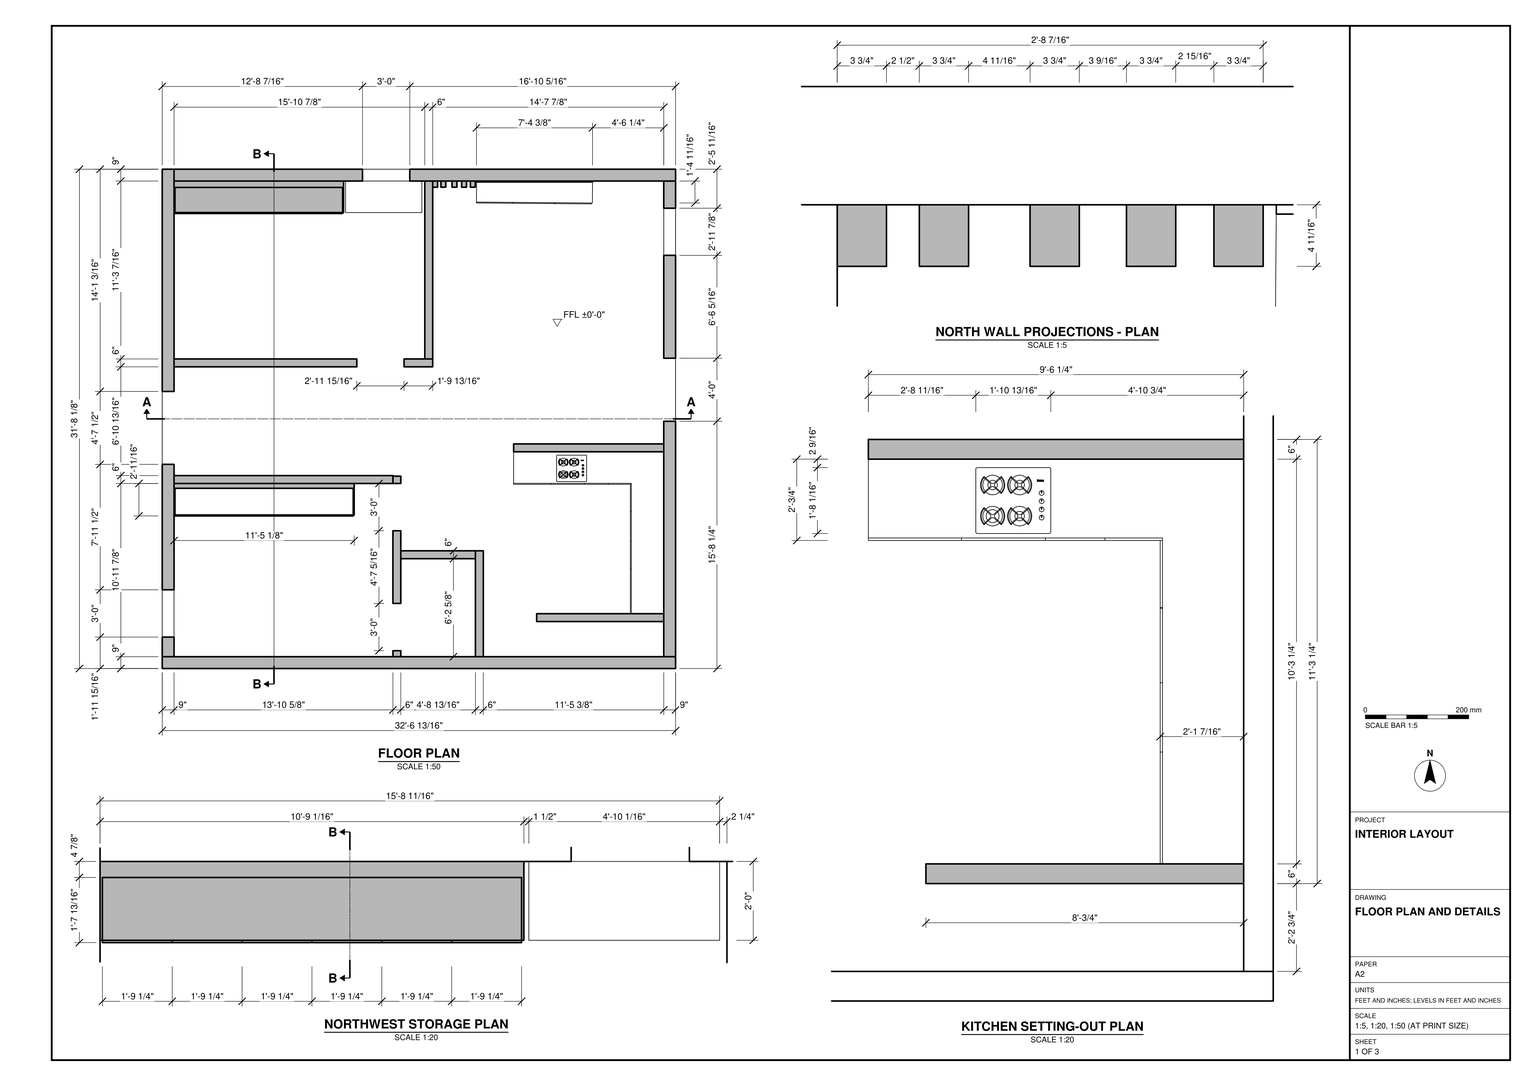
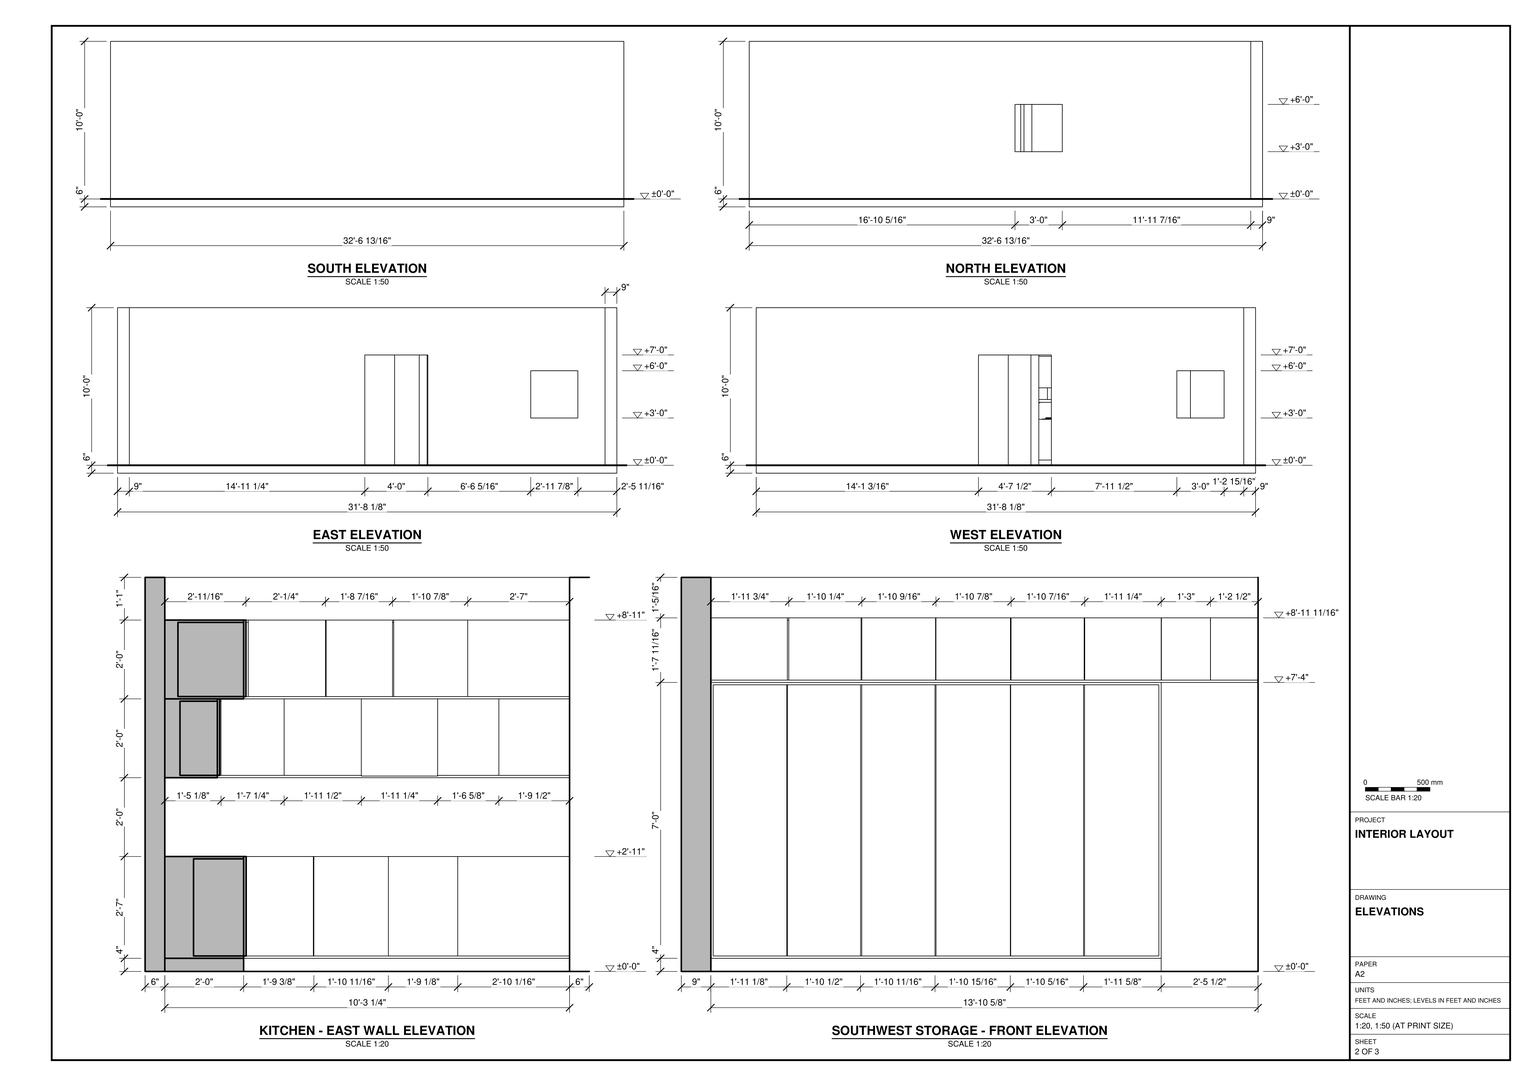
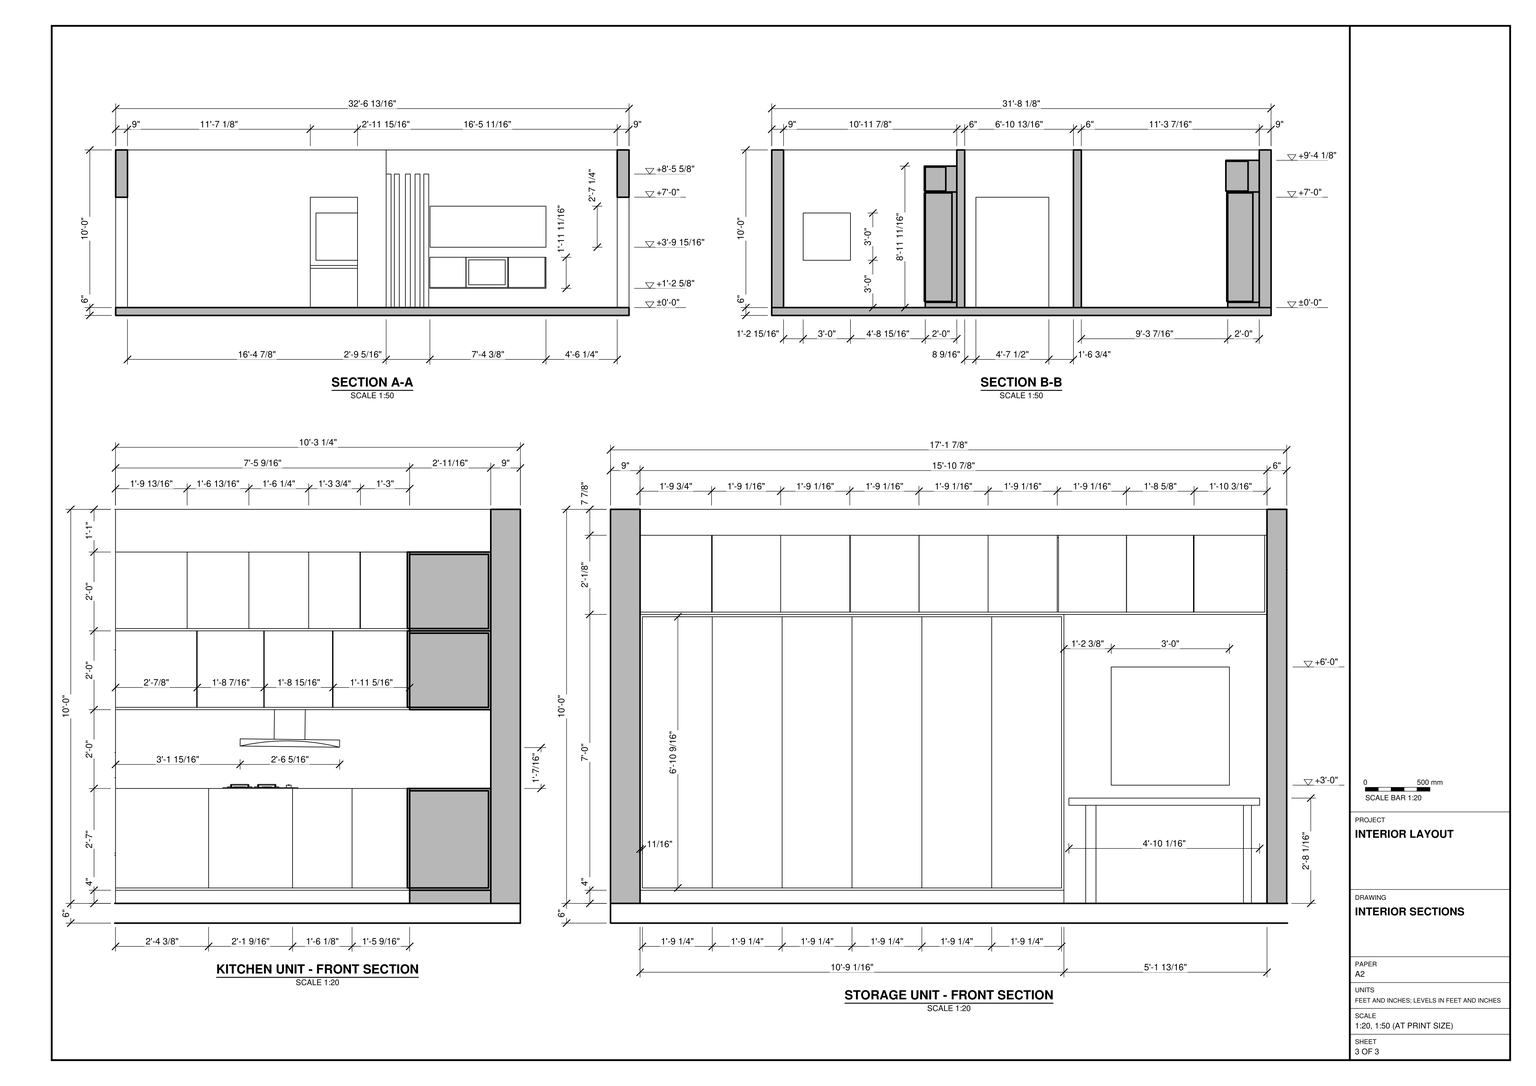
Build the interior in SketchUp from task_files/diagram_01.pdf. Work in feet and inches. Set the finished floor at ±0'-0". The overall dimensions are 32'-6 13/16" east to west, 31'-8 1/8" north to south and 10'-6" high, including the 6" floor slab below the finished floor.

Lay out the 9" perimeter walls and 6" interior partitions from the floor plan. Preserve the passage between the east and west doorway openings and the gaps that connect it to the rooms. Use the exterior elevations to set the window sills and heads; the south wall is uninterrupted.

Fit the northwest room with tall divided storage and a table beneath the window, with overhead cupboards extending across both. Build the southwest storage with its shorter bank of tall cupboards and longer overhead row. In the southeast kitchen, turn the worktop and cabinetry along the east wall. Follow the kitchen elevations for the plinths, cabinet divisions and two rows of upper cupboards. Place the cooktop on the transverse run with the extractor above it. On the north wall, use the projection detail and section A-A to position the vertical projections beside the raised cabinet and panel.

Keep shell elements and each furniture or joinery piece in separate groups or components, and use components for repeated parts. Decor, loose items and appliances may be any suitable library components. Save one SketchUp model as output_files/interior_with_fitted_storage_and_an_l_shaped_kitchen.skp.

# SketchUp Ruby script. Lengths in inches.
U = 1.inch
M = Sketchup.active_model
def pt(a) = Geom::Point3d.new(a.map { |v| v * U })
def face(e, loops, mat)
  f = e.add_face(loops[0].map { |a| pt(a) })
  loops[1..].each { |l| e.add_face(l.map { |a| pt(a) }).erase! }
  f.material = f.back_material = mat if mat
  f
end
# faces: each face lists its corners as indices into pts; further lists are holes
def faces(e, pts, list, mat = nil) = list.each { |f| face(e, (f[0].is_a?(Array) ? f : [f]).map { |l| l.map { |i| pts[i] } }, mat) }
# xy, xz, yz: faces in a plane at the given z, y or x. An outline is a flat list of corners, or four numbers for a rectangle; further outlines are holes
def ring(l) = l.size == 4 ? [[l[0], l[1]], [l[2], l[1]], [l[2], l[3]], [l[0], l[3]]] : l.each_slice(2).to_a
def flat(e, list, mat, &to3) = list.each { |f| face(e, (f[0].is_a?(Array) ? f : [f]).map { |l| ring(l).map { |u, v| to3.(u, v) } }, mat) }
def xy(e, z, list, mat = nil) = flat(e, list, mat) { |x, y| [x, y, z] }
def xz(e, y, list, mat = nil) = flat(e, list, mat) { |x, z| [x, y, z] }
def yz(e, x, list, mat = nil) = flat(e, list, mat) { |y, z| [x, y, z] }
def lines(e, pts, list) = list.each { |a, b| e.add_line(pt(pts[a]), pt(pts[b])) }
# prism: a flat outline (further loops are holes) pulled along v
def prism(e, loops, v, mat = nil)
  f = face(e, loops, mat); d = Geom::Vector3d.new(v.map { |x| x * U })
  f.pushpull(f.normal.samedirection?(d) ? d.length : -d.length)
end
def box(e, o, s, mat = nil) = prism(e, [[o, [o[0] + s[0], o[1], o[2]], [o[0] + s[0], o[1] + s[1], o[2]], [o[0], o[1] + s[1], o[2]]]], [0, 0, s[2]], mat)
def at(x, y, z, deg = 0) = Geom::Transformation.translation(pt([x, y, z])) * Geom::Transformation.rotation(ORIGIN, Z_AXIS, deg.degrees)
def axes(o, x, y, z) = Geom::Transformation.new([*x, 0, *y, 0, *z, 0, *pt(o).to_a, 1])
def part(name) = M.definitions.add(name)
# library, detail: a bought-in or finely detailed component or shape, given as its bounding box
def library(name, o, s) = part(name).tap { |d| box(d.entities, o, s) }
def detail(e, o, s) = box(e.add_group.entities, o, s)
def put(e, d, t, mat = nil) = e.add_instance(d, t).tap { |i| i.material = mat if mat }
def group(e, t, mat = nil) = e.add_group.tap { |g| g.transformation = t; g.material = mat if mat }.entities
root = M.entities
M.materials.add("[0011_Seashell]").color = [255, 245, 238]
M.materials.add("[0014_DarkSalmon]").color = [233, 150, 122]
M.materials.add("[Wood Floor]").color = [155, 105, 61]
M.materials.add("[Wood Veneer 01]").color = [120, 70, 37]
c1 = library("1-TABLE DE CUISSON CLC2",[-11.42,-10.04,0],[22.84,20.08,1.26])
c2 = library("5-HOTTE ASPIRANTE CLC2",[-15.16,-17.72,-0.29],[30.34,17.72,30.09])
c3 = part("Group\#44")
box(c3.entities,[0,0,0],[21.27,0.71,82.58])
c4 = part("Group\#45")
box(c4.entities,[0,0,0],[21.27,0.71,82.58])
c5 = part("Group\#62")
box(c5.entities,[0,-4.6875,0],[3.75,4.6875,101.64])
box(root,[356.38,119.78,4.71],[0.71,20.45,30.29])
box(root,[267.52,148.29,59.71],[24.71,0.71,23.29])
box(root,[326.36,140.29,83.71],[15.59,0.71,23.29])
box(root,[9,116.17,88.71],[23.29,0.71,18.97])
xy(root,4.71,[[9.71,116.17,32.11,116.88],[32.33,116.17,54.58,116.88],[54.94,116.17,77.25,116.88],[77.5625,116.17,100.18,116.88],[100.31,116.17,122.48,116.88],
  [122.8,116.17,145.42,116.88]])
xy(root,87.29,[[9.71,116.17,32.11,116.88],[32.33,116.17,54.58,116.88],[54.94,116.17,77.25,116.88],[77.5625,116.17,100.18,116.88],[100.31,116.17,122.48,116.88],
  [122.8,116.17,145.42,116.88]])
xy(root,88.71,[[9,345.71,30.76,346.42],[30.98,345.71,51.82,346.42],[51.82,345.71,72.87,346.42],[73.01,345.71,93.92,346.42],[93.97,345.71,114.98,346.42],
  [114.98,345.71,136.03,346.42],[136.41,345.71,157.08,346.42],[157.15,345.71,177.5,346.42],[177.7,345.71,199.19,346.42]])
xy(root,112.1,[[9,345.71,30.76,346.42],[30.98,345.71,51.82,346.42],[51.82,345.71,72.87,346.42],[73.01,345.71,93.92,346.42],[93.97,345.71,114.98,346.42],
  [114.98,345.71,136.03,346.42],[136.41,345.71,157.08,346.42],[157.15,345.71,177.5,346.42],[177.7,345.71,199.19,346.42]])
xz(root,116.17,[[9.71,4.71,32.11,87.29],[32.33,4.71,54.58,87.29],[54.94,4.71,77.25,87.29],[77.5625,4.71,100.18,87.29],[100.31,4.71,122.48,87.29],
  [122.8,4.71,145.42,87.29]],"[Wood Veneer 01]")
xz(root,116.88,[[9.71,4.71,32.11,87.29],[32.33,4.71,54.58,87.29],[54.94,4.71,77.25,87.29],[77.5625,4.71,100.18,87.29],[100.31,4.71,122.48,87.29],
  [122.8,4.71,145.42,87.29]])
xz(root,345.71,[[9,88.71,30.76,112.1],[30.98,88.71,51.82,112.1],[51.82,88.71,72.87,112.1],[73.01,88.71,93.92,112.1],[93.97,88.71,114.98,112.1],
  [114.98,88.71,136.03,112.1],[136.41,88.71,157.08,112.1],[157.15,88.71,177.5,112.1],[177.7,88.71,199.19,112.1]],"[0011_Seashell]")
xz(root,346.42,[[9,88.71,30.76,112.1],[30.98,88.71,51.82,112.1],[51.82,88.71,72.87,112.1],[93.97,88.71,114.98,112.1],[114.98,88.71,136.03,112.1],
  [177.7,88.71,199.19,112.1]])
yz(root,9,[[345.71,88.71,346.42,112.1]])
yz(root,9.71,[[116.17,4.71,116.88,87.29]])
yz(root,30.76,[[345.71,88.71,346.42,111.39],[345.71,111.39,346.42,112.1]])
yz(root,30.98,[[345.71,88.71,346.42,112.1]])
yz(root,32.11,[[116.17,4.71,116.88,87.29]])
yz(root,32.33,[[116.17,4.71,116.88,87.29]])
yz(root,51.82,[[345.71,88.71,346.42,112.1]])
yz(root,54.58,[[116.17,4.71,116.88,87.29]])
yz(root,54.94,[[116.17,4.71,116.88,87.29]])
yz(root,72.87,[[345.71,88.71,346.42,112.1]])
yz(root,73.01,[[345.71,88.71,346.42,112.1]])
yz(root,77.25,[[116.17,4.71,116.88,87.29]])
yz(root,77.5625,[[116.17,4.71,116.88,87.29]])
yz(root,93.92,[[345.71,88.71,346.42,112.1]])
yz(root,93.97,[[345.71,88.71,346.42,112.1]])
yz(root,100.18,[[116.17,4.71,116.88,87.29]])
yz(root,100.31,[[116.17,4.71,116.88,87.29]])
yz(root,114.98,[[345.71,88.71,346.42,112.1]])
yz(root,122.48,[[116.17,4.71,116.88,87.29]])
yz(root,122.8,[[116.17,4.71,116.88,87.29]])
yz(root,136.03,[[345.71,88.71,346.42,112.1]])
yz(root,136.41,[[345.71,88.71,346.42,112.1]])
yz(root,145.42,[[116.17,4.71,116.88,87.29]])
yz(root,157.08,[[345.71,88.71,346.42,112.1]])
yz(root,157.15,[[345.71,88.71,346.42,112.1]])
yz(root,177.5,[[345.71,88.71,346.42,112.1]])
yz(root,177.7,[[345.71,88.71,346.42,112.1]])
yz(root,199.19,[[345.71,88.71,346.42,112.1]])
p = [[9.71,346.42,111.39],[30.76,346.42,111.39],[30.98,346.42,111.39],[72.87,346.42,111.39],[73.01,346.42,111.39],[93.92,346.42,111.39],
  [93.97,346.42,111.39],[136.03,346.42,111.39],[136.41,346.42,111.39],[157.08,346.42,111.39],[157.15,346.42,111.39],[177.5,346.42,111.39],
  [177.7,346.42,111.39],[100.18,116.88,87.29],[100.31,116.88,87.29],[122.48,116.88,87.29],[122.8,116.88,87.29],[77.25,116.88,87.29],
  [77.5625,116.88,87.29],[54.58,116.88,87.29],[54.94,116.88,87.29],[32.11,116.88,87.29],[32.33,116.88,87.29]]
lines(root,p,[[0,1],[1,2],[3,4],[5,6],[7,8],[9,10],[11,12],[13,14],[15,16],[17,18],[19,20],[21,22]])
put(root,c1,at(311.65,152.39,35))
put(root,c2,axes([320.6,166.01,47.75],[0.99919,0,0],[0,1,0],[0,0,1]))
g1 = group(root,at(0,0,0))
box(g1,[0,0,0],[390.8,9,120])
g2 = group(root,at(0,9,0))
prism(g2,[[[0,371.125,0],[0,201.9375,0],[0,201.9375,84],[0,146.4375,84],[0,146.4375,0],[0,0,0],[0,0,120],[0,371.125,120]],[[0,50.9375,72],[0,14.9375,72],[0,14.9375,36],[0,50.9375,36]]],[9,0,0])
g3 = group(root,at(175.625,9,0))
prism(g3,[[[6,0,0],[6,4.57,0],[6,4.57,84],[6,40.57,84],[6,40.57,0],[6,95.88,0],[6,95.88,84],[6,131.88,84],[6,131.88,0],[6,137.45,0],[6,137.45,120],[6,0,120]]],[-6,0,0])
g4 = group(root,at(9,140.88,0))
box(g4,[0,0,0],[166.625,6,120])
g5 = group(root,at(238.43,9,0))
box(g5,[0,0,0],[6,80.625,120])
g6 = group(root,at(181.625,83.625,0))
box(g6,[0,0,0],[56.8,6,120])
g7 = group(root,at(381.8,9,0))
prism(g7,[[[9,0,0],[9,179.25,0],[9,179.25,84],[9,227.25,84],[9,227.25,0],[9,362.125,0],[9,362.125,120],[9,0,120]],[[9,305.5625,36],[9,305.5625,72],[9,341.4375,72],[9,341.4375,36]]],[-9,0,0])
g8 = group(root,at(9,371.125,0))
prism(g8,[[[0,0,0],[381.8,0,0],[381.8,0,120],[0,0,120]],[[179.46,0,72],[179.46,0,36],[143.46,0,36],[143.46,0,72]]],[0,9,0])
g9 = group(root,at(267.52,165,0))
box(g9,[0,0,0],[114.28,6,120])
g10 = group(root,at(199.9,235.68,0))
box(g10,[0,0,0],[6,135.45,120])
g11 = group(root,at(9,229.68,0))
prism(g11,[[[0,0,0],[139.15,0,0],[139.15,0,84],[175.1,0,84],[175.1,0,0],[196.9,0,0],[196.9,0,120],[0,0,120]]],[0,6,0])
g12 = group(root,at(0,0,-6))
box(g12,[0,0,0],[390.8,380.125,6])
g13 = group(root,at(285.05,35.75,0))
box(g13,[0,0,0],[96.75,6,120])
g14 = group(root,at(267.52,141,0))
prism(g14,[[[114.28,24,0],[114.28,-99.25,0],[89.57,-99.25,0],[89.57,0,0],[0,0,0],[0,24,0]]],[0,0,4])
g15 = group(root,at(267.52,141,4))
xy(g15,0,[[89.57,-99.25,89.57,0,0,0,0,24,114.28,24,114.28,-99.25]])
xy(g15,0.71,[[89.57,-99.25,113.57,-99.25,113.57,15.25,0.71,15.25,0.71,0,89.57,0]])
xy(g15,30.29,[[89.57,-99.25,89.57,0,0.71,0,0.71,15.25,113.57,15.25,113.57,-99.25]])
xy(g15,31,[[89.57,-99.25,114.28,-99.25,114.28,24,0,24,0,0,89.57,0]])
xz(g15,-99.25,[[89.57,0,114.28,0,114.28,31,89.57,31,89.57,30.29,113.57,30.29,113.57,0.71,89.57,0.71]])
xz(g15,0,[[0,0,89.57,0,89.57,0.71,0.71,0.71,0.71,30.29,89.57,30.29,89.57,31,0,31]])
xz(g15,15.25,[[0.71,0.71,113.57,30.29]])
xz(g15,24,[[0,0,114.28,31]])
yz(g15,0,[[0,0,24,31]])
yz(g15,0.71,[[0,0.71,15.25,30.29]])
yz(g15,89.57,[[-99.25,0,0,0.71],[-99.25,30.29,0,31]])
yz(g15,113.57,[[-99.25,0.71,15.25,30.29]])
yz(g15,114.28,[[-99.25,0,24,31]])
g16 = group(root,at(267.52,140.23,4.71))
box(g16,[0,0,0],[28.35,0.77,30.29])
g17 = group(root,at(295.87,140.23,4.71))
box(g17,[0,0,0],[25.5625,0.77,30.29])
g18 = group(root,at(321.43,140.23,4.71))
box(g18,[0,0,0],[18.125,0.77,30.29])
g19 = group(root,at(339.56,140.23,4.71))
box(g19,[0,0,0],[17.53,0.77,30.29])
g20 = group(root,at(356.38,96.92,4.71))
box(g20,[0,0,0],[0.71,22.69,30.29])
g21 = group(root,at(356.38,75.8,4.71))
box(g21,[0,0,0],[0.71,21.11,30.29])
g22 = group(root,at(356.38,41.75,4.71))
box(g22,[0,0,0],[0.71,34.05,30.29])
g23 = group(root,at(267.52,165,59))
xy(g23,0,[[89.57,-123.25,89.57,-16,0,-16,0,0,114.28,0,114.28,-123.25]])
xy(g23,0.71,[[89.57,-123.25,113.57,-123.25,113.57,-4.625,0.71,-4.625,0.71,-16,89.57,-16]])
xy(g23,23.29,[[89.57,-123.25,89.57,-16,0.71,-16,0.71,-4.625,113.57,-4.625,113.57,-123.25]])
xy(g23,24,[[89.57,-123.25,114.28,-123.25,114.28,0,0,0,0,-16,89.57,-16]])
xz(g23,-123.25,[[89.57,0,114.28,0,114.28,24,89.57,24,89.57,23.29,113.57,23.29,113.57,0.71,89.57,0.71]])
xz(g23,-16,[[0,0,89.57,0,89.57,0.71,0.71,0.71,0.71,23.29,89.57,23.29,89.57,24,0,24]])
xz(g23,-4.625,[[0.71,0.71,113.57,23.29]])
xz(g23,0,[[0,0,114.28,24]])
yz(g23,0,[[-16,0,0,24]])
yz(g23,0.71,[[-16,0.71,-4.625,23.29]])
yz(g23,89.57,[[-123.25,0,-16,0.71],[-123.25,23.29,-16,24]])
yz(g23,113.57,[[-123.25,0.71,-4.625,23.29]])
yz(g23,114.28,[[-123.25,0,0,24]])
g24 = group(root,at(292.41,148.29,59.71))
box(g24,[0,0,0],[20.25,0.71,23.29])
g25 = group(root,at(312.82,148.29,59.71))
box(g25,[0,0,0],[20.76,0.71,23.29])
g26 = group(root,at(333.77,148.29,59.71))
box(g26,[0,0,0],[23.32,0.71,23.29])
g27 = group(root,at(356.38,128.66,59.71))
box(g27,[0,0,0],[0.71,19.22,23.29])
g28 = group(root,at(356.38,105.17,59.71))
box(g28,[0,0,0],[0.71,23.5,23.29])
g29 = group(root,at(356.38,81.92,59))
box(g29,[0,0,0.5],[0.71,23.25,23.5])
g30 = group(root,at(356.38,63.28,59.71))
box(g30,[0,0,0],[0.71,18.64,23.29])
g31 = group(root,at(356.38,41.75,59.71))
box(g31,[0,0,0],[0.71,21.53,23.29])
g32 = group(root,at(267.52,165,83))
xy(g32,0,[[89.57,-123.25,89.57,-24,0,-24,0,0,114.28,0,114.28,-123.25]])
xy(g32,0.71,[[89.57,-123.25,113.57,-123.25,113.57,-4,0.71,-4,0.71,-24,89.57,-24]])
xy(g32,23.29,[[89.57,-123.25,89.57,-24,0.71,-24,0.71,-4,113.57,-4,113.57,-123.25]])
xy(g32,24,[[89.57,-123.25,114.28,-123.25,114.28,0,0,0,0,-24,89.57,-24]])
xz(g32,-123.25,[[89.57,0,114.28,0,114.28,24,89.57,24,89.57,23.29,113.57,23.29,113.57,0.71,89.57,0.71]])
xz(g32,-24,[[0,0,89.57,0,89.57,0.71,0.71,0.71,0.71,23.29,89.57,23.29,89.57,24,0,24]])
xz(g32,-4,[[0.71,0.71,113.57,23.29]])
xz(g32,0,[[0,0,114.28,24]])
yz(g32,0,[[-24,0,0,24]])
yz(g32,0.71,[[-24,0.71,-4,23.29]])
yz(g32,89.57,[[-123.25,0,-24,0.71],[-123.25,23.29,-24,24]])
yz(g32,113.57,[[-123.25,0.71,-4,23.29]])
yz(g32,114.28,[[-123.25,0,0,24]])
g33 = group(root,at(267.52,140.29,83.71))
box(g33,[0,0,0],[21.81,0.71,23.29])
g34 = group(root,at(289.34,140.29,83.71))
box(g34,[0,0,0],[18.8,0.71,23.29])
g35 = group(root,at(308.13,140.29,83.71))
box(g35,[0,0,0],[18.22,0.71,23.29])
g36 = group(root,at(342.49,140.29,83.71))
box(g36,[-0.375,0,0],[14.98,0.71,23.29])
g37 = group(root,at(356.38,116.07,83.71))
box(g37,[0,0,0],[0.71,23.53,23.29])
g38 = group(root,at(356.38,95.65,83.71))
box(g38,[0,0,0],[0.71,20.21,23.29])
g39 = group(root,at(356.38,76.76,83.71))
box(g39,[0,-4,0],[0.71,22.53,23.29])
g40 = group(root,at(356.38,41.75,83.71))
box(g40,[0,0,0],[0.71,31.01,23.29])
g41 = group(root,at(9,347.125,0))
box(g41,[0,0,0],[129.0625,24,4])
g42 = group(root,at(9,347.125,4))
xy(g42,0,[[0,0,129.0625,24]])
xy(g42,0.71,[[0.71,0,128.35,19.125]])
xy(g42,83.29,[[0.71,0,128.35,19.125]])
xy(g42,84,[[0,0,129.0625,24]])
xz(g42,0,[[[0,0,129.0625,84],[0.71,0.71,128.35,83.29]]])
xz(g42,19.125,[[0.71,0.71,128.35,83.29]])
xz(g42,24,[[0,0,129.0625,84]])
yz(g42,0,[[0,0,24,84]])
yz(g42,0.71,[[0,0.71,19.125,83.29]])
yz(g42,128.35,[[0,0.71,19.125,83.29]])
yz(g42,129.0625,[[0,0,24,84]])
put(root,c3,at(116.08,346.42,4.71),"[0014_DarkSalmon]")
put(root,c3,at(94.81,346.42,4.71),"[0014_DarkSalmon]")
put(root,c3,at(73.53,346.42,4.71),"[0014_DarkSalmon]")
put(root,c4,at(52.26,346.42,4.71),"[0014_DarkSalmon]")
put(root,c4,at(30.98,346.42,4.71),"[0014_DarkSalmon]")
put(root,c4,at(9.71,346.42,4.71),"[0014_DarkSalmon]")
g43 = group(root,at(9,371.125,88))
xy(g43,0,[[0,-24.71,190.9,0]])
xy(g43,0.71,[[0.71,-24.71,190.19,-8.52]])
xy(g43,23.39,[[0.71,-24.71,190.19,-8.52]])
xy(g43,24.1,[[0,-24.71,190.9,0]])
xz(g43,-24.71,[[[0,0,190.9,24.1],[0.71,0.71,190.19,23.39]]])
xz(g43,-8.52,[[0.71,0.71,190.19,23.39]])
xz(g43,0,[[0,0,190.9,24.1]])
yz(g43,0,[[-24.71,0,0,24.1]])
yz(g43,0.71,[[-24.71,0.71,-8.52,23.39]])
yz(g43,190.19,[[-24.71,0.71,-8.52,23.39]])
yz(g43,190.9,[[-24.71,0,0,24.1]])
g44 = group(root,at(139.58,371.125,29.875),"[Wood Veneer 01]")
xy(g44,0,[[0,-24,58.09,0]],"[Wood Floor]")
xy(g44,2.1875,[[0,-24,58.09,0]],"[Wood Veneer 01]")
xz(g44,-24,[[0,0,58.09,2.1875]],"[Wood Veneer 01]")
xz(g44,0,[[0,0,58.09,2.1875]],"[Wood Floor]")
yz(g44,0,[[-24,0,0,2.1875]],"[Wood Floor]")
yz(g44,58.09,[[-24,0,0,2.1875]],"[Wood Floor]")
g45 = group(root,at(9,116.88,0))
box(g45,[0,0,0],[137.125,24,4])
g46 = group(root,at(9,116.88,4))
xy(g46,0,[[0,0,137.125,24]])
xy(g46,0.71,[[0.71,0,136.42,20.3125]])
xy(g46,83.29,[[0.71,0,136.42,20.3125]])
xy(g46,84,[[0,0,137.125,24]])
xz(g46,0,[[[0,0,137.125,84],[0.71,0.71,136.42,83.29]]])
xz(g46,20.3125,[[0.71,0.71,136.42,83.29]])
xz(g46,24,[[0,0,137.125,84]])
yz(g46,0,[[0,0,24,84]])
yz(g46,0.71,[[0,0.71,20.3125,83.29]])
yz(g46,136.42,[[0,0.71,20.3125,83.29]])
yz(g46,137.125,[[0,0,24,84]])
g47 = group(root,at(9,140.88,88))
xy(g47,0,[[0,-24,166.625,0]])
xy(g47,0.71,[[0.71,-24,165.92,-8.375]])
xy(g47,18.97,[[0.71,-24,165.92,-8.375]])
xy(g47,19.68,[[0,-24,166.625,0]])
xz(g47,-24,[[[0,0,166.625,19.68],[0.71,0.71,165.92,18.97]]])
xz(g47,-8.375,[[0.71,0.71,165.92,18.97]])
xz(g47,0,[[0,0,166.625,19.68]])
yz(g47,0,[[-24,0,0,19.68]])
yz(g47,0.71,[[-24,0.71,-8.375,18.97]])
yz(g47,165.92,[[-24,0.71,-8.375,18.97]])
yz(g47,166.625,[[-24,0,0,19.68]])
g48 = group(root,at(32.73,116.17,88.71))
box(g48,[0,0,0],[22,0.71,18.97])
g49 = group(root,at(54.98,116.17,88.71))
box(g49,[0,0,0],[22.44,0.71,18.97])
g50 = group(root,at(100.41,116.17,88.71))
box(g50,[0,0,0],[22.25,0.71,18.97])
g51 = group(root,at(77.54,116.17,88.71))
box(g51,[0,0,0],[22.6875,0.71,18.97])
g52 = group(root,at(122.85,116.17,88.71))
box(g52,[0,0,0],[23.27,0.71,18.97])
g53 = group(root,at(146.51,116.17,88.71))
box(g53,[-0.3125,0,0],[14.93,0.71,18.97])
g54 = group(root,at(161.15,116.17,88.71))
box(g54,[0,0,0],[14.48,0.71,18.97])
g55 = group(root,at(239.33,371.125,45.93))
box(g55,[0,-0.71,0],[88.25,0.71,31.25])
g56 = group(root,at(239.33,370.42,14.625))
xy(g56,0,[[88.12,-16,-0.13,-15.29,0,0.71,88.25,0]])
xy(g56,0.71,[[87.41,-15.99,87.53,-1.81,0.69,-1.11,0.58,-15.3]])
xy(g56,22.97,[[87.41,-15.99,0.58,-15.3,0.69,-1.11,87.53,-1.81]])
xy(g56,23.68,[[88.12,-16,88.25,0,0,0.71,-0.13,-15.29]])
p = [[-0.13,-15.29,0],[88.12,-16,0],[88.12,-16,23.68],[-0.13,-15.29,23.68],[87.41,-15.99,0.71],[0.58,-15.3,0.71],
  [0.58,-15.3,22.97],[87.41,-15.99,22.97],[88.25,0,0],[88.25,0,23.68],[0,0.71,23.68],[0,0.71,0],
  [87.53,-1.81,22.97],[87.53,-1.81,0.71],[0.69,-1.11,0.71],[0.69,-1.11,22.97]]
faces(g56,p,[[[0,1,2,3],[4,5,6,7]],[8,9,2,1],[10,11,0,3],[8,11,10,9],[4,7,12,13],[6,5,14,15],[14,13,12,15]])
g57 = group(root,at(239.19,354.2,15.33))
prism(g57,[[[0.01,0.93,0],[27.41,0.71,0],[27.41,0,0],[0,0.22,0]]],[0,0,22.97])
g58 = group(root,at(266.77,353.94,15.33))
prism(g58,[[[0,0.25,0],[31.75,0,0],[31.75,0,22.97],[0,0.25,22.97]],[[29.75,0.02,20.97],[29.75,0.02,2],[2,0.24,2],[2,0.24,20.97]]],[0.01,0.71,0])
g59 = group(root,at(298.93,353.71,15.33))
prism(g59,[[[0.01,0.93,0],[27.8125,0.71,0],[27.81,0,0],[0,0.22,0]]],[0,0,22.97])
put(root,c5,at(212.15,371.125,0))
put(root,c5,at(205.9,371.125,0))
put(root,c5,at(220.58,371.125,0))
put(root,c5,at(227.92,371.125,0))
put(root,c5,at(234.58,371.125,0))
g60 = group(root,at(144.7,347.125,29.875))
xy(g60,0,[[0,0,3.125,24]])
g61 = group(root,at(144.7,371.125,0))
xz(g61,0,[[0,0,3.125,29.875]])
g62 = group(root,at(192.73,371.125,0))
xz(g62,0,[[0,0,2.4375,29.875]])
g63 = group(root,at(192.73,347.125,29.875))
xy(g63,0,[[0,0,2.05,24]])
